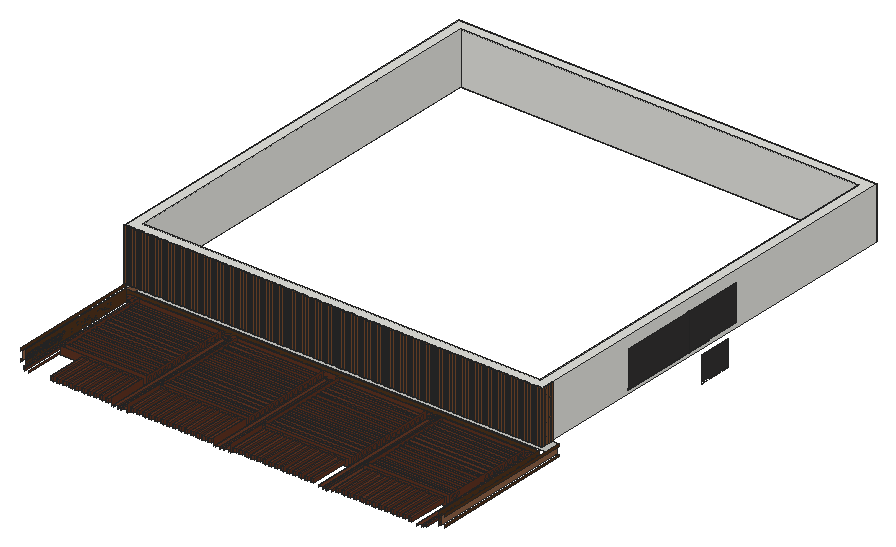
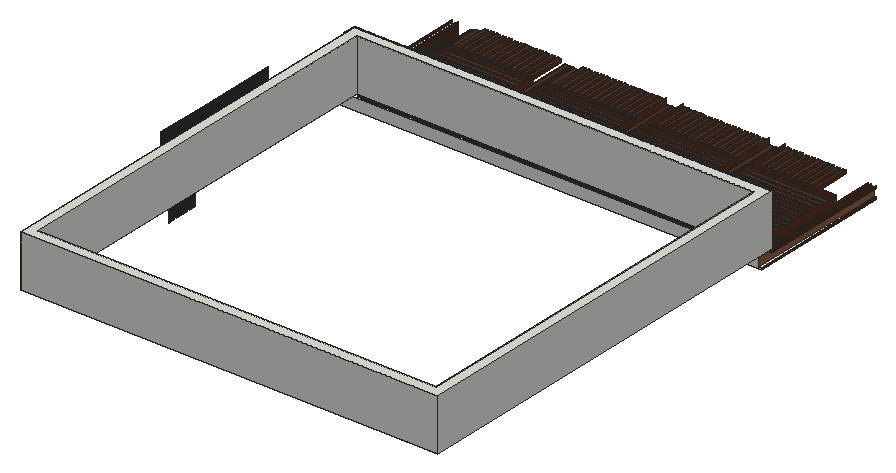
# SketchUp Ruby script. Lengths in inches.
U = 1.inch
M = Sketchup.active_model
def pt(a) = Geom::Point3d.new(a.map { |v| v * U })
def face(e, loops, mat)
  f = e.add_face(loops[0].map { |a| pt(a) })
  loops[1..].each { |l| e.add_face(l.map { |a| pt(a) }).erase! }
  f.material = f.back_material = mat if mat
  f
end
# faces: each face lists its corners as indices into pts; further lists are holes
def faces(e, pts, list, mat = nil) = list.each { |f| face(e, (f[0].is_a?(Array) ? f : [f]).map { |l| l.map { |i| pts[i] } }, mat) }
# xy, xz, yz: faces in a plane at the given z, y or x. An outline is a flat list of corners, or four numbers for a rectangle; further outlines are holes
def ring(l) = l.size == 4 ? [[l[0], l[1]], [l[2], l[1]], [l[2], l[3]], [l[0], l[3]]] : l.each_slice(2).to_a
def flat(e, list, mat, &to3) = list.each { |f| face(e, (f[0].is_a?(Array) ? f : [f]).map { |l| ring(l).map { |u, v| to3.(u, v) } }, mat) }
def xy(e, z, list, mat = nil) = flat(e, list, mat) { |x, y| [x, y, z] }
def xz(e, y, list, mat = nil) = flat(e, list, mat) { |x, z| [x, y, z] }
def yz(e, x, list, mat = nil) = flat(e, list, mat) { |y, z| [x, y, z] }
def lines(e, pts, list) = list.each { |a, b| e.add_line(pt(pts[a]), pt(pts[b])) }
# prism: a flat outline (further loops are holes) pulled along v
def prism(e, loops, v, mat = nil)
  f = face(e, loops, mat); d = Geom::Vector3d.new(v.map { |x| x * U })
  f.pushpull(f.normal.samedirection?(d) ? d.length : -d.length)
end
def box(e, o, s, mat = nil) = prism(e, [[o, [o[0] + s[0], o[1], o[2]], [o[0] + s[0], o[1] + s[1], o[2]], [o[0], o[1] + s[1], o[2]]]], [0, 0, s[2]], mat)
def at(x, y, z, deg = 0) = Geom::Transformation.translation(pt([x, y, z])) * Geom::Transformation.rotation(ORIGIN, Z_AXIS, deg.degrees)
def axes(o, x, y, z) = Geom::Transformation.new([*x, 0, *y, 0, *z, 0, *pt(o).to_a, 1])
def part(name) = M.definitions.add(name)
# library, detail: a bought-in or finely detailed component or shape, given as its bounding box
def library(name, o, s) = part(name).tap { |d| box(d.entities, o, s) }
def detail(e, o, s) = box(e.add_group.entities, o, s)
def put(e, d, t, mat = nil) = e.add_instance(d, t).tap { |i| i.material = mat if mat }
def group(e, t, mat = nil) = e.add_group.tap { |g| g.transformation = t; g.material = mat if mat }.entities
root = M.entities
M.materials.add("1799 AP 8574 BURNISHED CARAMEL").color = [140, 96, 69]
M.materials.add("1816 AP K197 Dark Kaapi-N").color = [79, 50, 27]
M.materials.add("[Granite Dark Gray]").color = [51, 50, 50]
M.materials.add("[Wood Cherry Original]").color = [118, 74, 44]
M.materials.add("[Wood Cherry Original]1").color = [93, 50, 33]
c1 = part("3")
box(c1.entities,[0,0,0],[3,2,36])
c2 = part("2")
box(c2.entities,[0,0,0],[3,2,75.23])
c3 = part("Group247\#1")
box(c3.entities,[-192,-24,0],[2.5,48,0.5])
c4 = part("Group248\#1")
box(c4.entities,[-189,-24,0],[2.5,48,0.5])
c5 = part("Group249\#1")
box(c5.entities,[-186,-24,0],[2.5,48,0.5])
c6 = part("Group250\#1")
box(c6.entities,[-183,-24,0],[2.5,48,0.5])
c7 = part("Group251\#1")
box(c7.entities,[-180,-24,0],[2.5,48,0.5])
c8 = part("Group252\#1")
box(c8.entities,[-177,-24,0],[2.5,48,0.5])
c9 = part("Group253\#1")
box(c9.entities,[-174,-24,0],[2.5,48,0.5])
c10 = part("Group254\#1")
box(c10.entities,[-171,-24,0],[2.5,48,0.5])
c11 = part("Group255\#1")
box(c11.entities,[-168,-24,0],[2.5,48,0.5])
c12 = part("Group256\#1")
box(c12.entities,[-165,-24,0],[2.5,48,0.5])
c13 = part("Group257\#1")
box(c13.entities,[-162,-24,0],[2.5,48,0.5])
c14 = part("Group258\#1")
box(c14.entities,[-159,-24,0],[2.5,48,0.5])
c15 = part("Group259\#1")
box(c15.entities,[-156,-24,0],[2.5,48,0.5])
c16 = part("Group260\#1")
box(c16.entities,[-153,-24,0],[2.5,48,0.5])
c17 = part("Group261\#1")
box(c17.entities,[-150,-24,0],[2.5,48,0.5])
c18 = part("Group262\#1")
box(c18.entities,[-147,-24,0],[2.5,48,0.5])
c19 = part("Group263\#1")
box(c19.entities,[-144,-24,0],[2.5,48,0.5])
c20 = part("Group264\#1")
box(c20.entities,[-141,-24,0],[2.5,48,0.5])
c21 = part("Group265\#1")
box(c21.entities,[-138,-24,0],[2.5,48,0.5])
c22 = part("Group266\#1")
box(c22.entities,[-135,-24,0],[2.5,48,0.5])
c23 = part("Group267\#1")
box(c23.entities,[-132,-24,0],[2.5,48,0.5])
c24 = part("Group268\#1")
box(c24.entities,[-129,-24,0],[2.5,48,0.5])
c25 = part("Group269\#1")
box(c25.entities,[-126,-24,0],[2.5,48,0.5])
c26 = part("Group270\#1")
box(c26.entities,[-123,-24,0],[2.5,48,0.5])
c27 = part("Group271\#1")
box(c27.entities,[-120,-24,0],[2.5,48,0.5])
c28 = part("Group272\#1")
box(c28.entities,[-117,-24,0],[2.5,48,0.5])
c29 = part("Group273\#1")
box(c29.entities,[-114,-24,0],[2.5,48,0.5])
c30 = part("Group274\#1")
box(c30.entities,[-111,-24,0],[2.5,48,0.5])
c31 = part("Group275\#1")
box(c31.entities,[-108,-24,0],[2.5,48,0.5])
c32 = part("Group276\#1")
box(c32.entities,[-105,-24,0],[2.5,48,0.5])
c33 = part("Group277\#1")
box(c33.entities,[-102,-24,0],[2.5,48,0.5])
c34 = part("Group278\#1")
box(c34.entities,[-99,-24,0],[2.5,48,0.5])
c35 = part("Group279\#1")
box(c35.entities,[-96,-24,0],[2.5,48,0.5])
c36 = part("Group280\#1")
box(c36.entities,[-93,-24,0],[2.5,48,0.5])
c37 = part("Group281\#1")
box(c37.entities,[-90,-24,0],[2.5,48,0.5])
c38 = part("Group282\#1")
box(c38.entities,[-87,-24,0],[2.5,48,0.5])
c39 = part("Group283\#1")
box(c39.entities,[-84,-24,0],[2.5,48,0.5])
c40 = part("Group284\#1")
box(c40.entities,[-81,-24,0],[2.5,48,0.5])
c41 = part("Group285\#1")
box(c41.entities,[-78,-24,0],[2.5,48,0.5])
c42 = part("Group286\#1")
box(c42.entities,[-75,-24,0],[2.5,48,0.5])
c43 = part("Group287\#1")
box(c43.entities,[-72,-24,0],[2.5,48,0.5])
c44 = part("Group288\#1")
box(c44.entities,[-69,-24,0],[2.5,48,0.5])
c45 = part("Group289\#1")
box(c45.entities,[-66,-24,0],[2.5,48,0.5])
c46 = part("Group290\#1")
box(c46.entities,[-63,-24,0],[2.5,48,0.5])
c47 = part("Group291\#1")
box(c47.entities,[-60,-24,0],[2.5,48,0.5])
c48 = part("Group292\#1")
box(c48.entities,[-57,-24,0],[2.5,48,0.5])
c49 = part("Group293\#1")
box(c49.entities,[-54,-24,0],[2.5,48,0.5])
c50 = part("Group294\#1")
box(c50.entities,[-51,-24,0],[2.5,48,0.5])
c51 = part("Group295\#1")
box(c51.entities,[-48,-24,0],[2.5,48,0.5])
c52 = part("Group296\#1")
box(c52.entities,[-45,-24,0],[2.5,48,0.5])
c53 = part("Group297\#1")
box(c53.entities,[-42,-24,0],[2.5,48,0.5])
c54 = part("Group298\#1")
box(c54.entities,[-39,-24,0],[2.5,48,0.5])
c55 = part("Group299\#1")
box(c55.entities,[-36,-24,0],[2.5,48,0.5])
c56 = part("Group300\#1")
box(c56.entities,[-33,-24,0],[2.5,48,0.5])
c57 = part("Group301\#1")
box(c57.entities,[-30,-24,0],[2.5,48,0.5])
c58 = part("Group302\#1")
box(c58.entities,[-27,-24,0],[2.5,48,0.5])
c59 = part("Group303\#1")
box(c59.entities,[-24,-24,0],[2.5,48,0.5])
c60 = part("Group304\#1")
box(c60.entities,[-21,-24,0],[2.5,48,0.5])
c61 = part("Group305\#1")
box(c61.entities,[-18,-24,0],[2.5,48,0.5])
c62 = part("Group306\#1")
box(c62.entities,[-15,-24,0],[2.5,48,0.5])
c63 = part("Group307\#1")
box(c63.entities,[-12,-24,0],[2.5,48,0.5])
c64 = part("Group308\#1")
box(c64.entities,[-9,-24,0],[2.5,48,0.5])
c65 = part("Group309\#1")
box(c65.entities,[-6,-24,0],[2.5,48,0.5])
c66 = part("Group310\#1")
box(c66.entities,[-3,-24,0],[2.5,48,0.5])
c67 = part("Group311\#1")
box(c67.entities,[0,-24,0],[2.5,48,0.5])
c68 = part("Group312\#1")
box(c68.entities,[3,-24,0],[2.5,48,0.5])
c69 = part("Group313\#1")
box(c69.entities,[6,-24,0],[2.5,48,0.5])
c70 = part("Group314\#1")
box(c70.entities,[9,-24,0],[2.5,48,0.5])
c71 = part("Group315\#1")
box(c71.entities,[12,-24,0],[2.5,48,0.5])
c72 = part("Group316\#1")
box(c72.entities,[15,-24,0],[2.5,48,0.5])
c73 = part("Group317\#1")
box(c73.entities,[18,-24,0],[2.5,48,0.5])
c74 = part("Group318\#1")
box(c74.entities,[21,-24,0],[2.5,48,0.5])
c75 = part("Group319\#1")
box(c75.entities,[24,-24,0],[2.5,48,0.5])
c76 = part("Group320\#1")
box(c76.entities,[27,-24,0],[2.5,48,0.5])
c77 = part("Group321\#1")
box(c77.entities,[30,-24,0],[2.5,48,0.5])
c78 = part("Group322\#1")
box(c78.entities,[33,-24,0],[2.5,48,0.5])
c79 = part("Group323\#1")
box(c79.entities,[36,-24,0],[2.5,48,0.5])
c80 = part("Group324\#1")
box(c80.entities,[39,-24,0],[2.5,48,0.5])
c81 = part("Group325\#1")
box(c81.entities,[42,-24,0],[2.5,48,0.5])
c82 = part("Group326\#1")
box(c82.entities,[45,-24,0],[2.5,48,0.5])
c83 = part("Group327\#1")
box(c83.entities,[48,-24,0],[2.5,48,0.5])
c84 = part("Group328\#1")
box(c84.entities,[51,-24,0],[2.5,48,0.5])
c85 = part("Group329\#1")
box(c85.entities,[54,-24,0],[2.5,48,0.5])
c86 = part("Group330\#1")
box(c86.entities,[57,-24,0],[2.5,48,0.5])
c87 = part("Group331\#1")
box(c87.entities,[60,-24,0],[2.5,48,0.5])
c88 = part("Group332\#1")
box(c88.entities,[63,-24,0],[2.5,48,0.5])
c89 = part("Group333\#1")
box(c89.entities,[66,-24,0],[2.5,48,0.5])
c90 = part("Group334\#1")
box(c90.entities,[69,-24,0],[2.5,48,0.5])
c91 = part("Group335\#1")
box(c91.entities,[72,-24,0],[2.5,48,0.5])
c92 = part("Group336\#1")
box(c92.entities,[75,-24,0],[2.5,48,0.5])
c93 = part("Group337\#1")
box(c93.entities,[78,-24,0],[2.5,48,0.5])
c94 = part("Group338\#1")
box(c94.entities,[81,-24,0],[2.5,48,0.5])
c95 = part("Group339\#1")
box(c95.entities,[84,-24,0],[2.5,48,0.5])
c96 = part("Group340\#1")
box(c96.entities,[87,-24,0],[2.5,48,0.5])
c97 = part("Group341\#1")
box(c97.entities,[90,-24,0],[2.5,48,0.5])
c98 = part("Group342\#1")
box(c98.entities,[93,-24,0],[2.5,48,0.5])
c99 = part("Group343\#1")
box(c99.entities,[96,-24,0],[2.5,48,0.5])
c100 = part("Group344\#1")
box(c100.entities,[99,-24,0],[2.5,48,0.5])
c101 = part("Group345\#1")
box(c101.entities,[102,-24,0],[2.5,48,0.5])
c102 = part("Group346\#1")
box(c102.entities,[105,-24,0],[2.5,48,0.5])
c103 = part("Group347\#1")
box(c103.entities,[108,-24,0],[2.5,48,0.5])
c104 = part("Group348\#1")
box(c104.entities,[111,-24,0],[2.5,48,0.5])
c105 = part("Group349\#1")
box(c105.entities,[114,-24,0],[2.5,48,0.5])
c106 = part("Group350\#1")
box(c106.entities,[117,-24,0],[2.5,48,0.5])
c107 = part("Group351\#1")
box(c107.entities,[120,-24,0],[2.5,48,0.5])
c108 = part("Group352\#1")
box(c108.entities,[123,-24,0],[2.5,48,0.5])
c109 = part("Group353\#1")
box(c109.entities,[126,-24,0],[2.5,48,0.5])
c110 = part("Group354\#1")
box(c110.entities,[129,-24,0],[2.5,48,0.5])
c111 = part("Group355\#1")
box(c111.entities,[132,-24,0],[2.5,48,0.5])
c112 = part("Group356\#1")
box(c112.entities,[135,-24,0],[2.5,48,0.5])
c113 = part("Group357\#1")
box(c113.entities,[138,-24,0],[2.5,48,0.5])
c114 = part("Group358\#1")
box(c114.entities,[141,-24,0],[2.5,48,0.5])
c115 = part("Group359\#1")
box(c115.entities,[144,-24,0],[2.5,48,0.5])
c116 = part("Group360\#1")
box(c116.entities,[147,-24,0],[2.5,48,0.5])
c117 = part("Group361\#1")
box(c117.entities,[150,-24,0],[2.5,48,0.5])
c118 = part("Group362\#1")
box(c118.entities,[153,-24,0],[2.5,48,0.5])
c119 = part("Group363\#1")
box(c119.entities,[156,-24,0],[2.5,48,0.5])
c120 = part("Group364\#1")
box(c120.entities,[159,-24,0],[2.5,48,0.5])
c121 = part("Group365\#1")
box(c121.entities,[162,-24,0],[2.5,48,0.5])
c122 = part("Group366\#1")
box(c122.entities,[165,-24,0],[2.5,48,0.5])
c123 = part("Group367\#1")
box(c123.entities,[168,-24,0],[2.5,48,0.5])
c124 = part("Group368\#1")
box(c124.entities,[171,-24,0],[2.5,48,0.5])
c125 = part("Group369\#1")
box(c125.entities,[174,-24,0],[2.5,48,0.5])
c126 = part("Group370\#1")
box(c126.entities,[177,-24,0],[2.5,48,0.5])
c127 = part("Group371\#1")
box(c127.entities,[180,-24,0],[2.5,48,0.5])
c128 = part("Group372\#1")
box(c128.entities,[183,-24,0],[2.5,48,0.5])
c129 = part("Group373\#1")
box(c129.entities,[186,-24,0],[2.5,48,0.5])
c130 = part("Group374\#1")
box(c130.entities,[189,-24,0],[2.5,48,0.5])
c131 = part("Group245\#1")
put(c131.entities,c3,at(0,0,0))
put(c131.entities,c4,at(0,0,0))
put(c131.entities,c5,at(0,0,0))
put(c131.entities,c6,at(0,0,0))
put(c131.entities,c7,at(0,0,0))
put(c131.entities,c8,at(0,0,0))
put(c131.entities,c9,at(0,0,0))
put(c131.entities,c10,at(0,0,0))
put(c131.entities,c11,at(0,0,0))
put(c131.entities,c12,at(0,0,0))
put(c131.entities,c13,at(0,0,0))
put(c131.entities,c14,at(0,0,0))
put(c131.entities,c15,at(0,0,0))
put(c131.entities,c16,at(0,0,0))
put(c131.entities,c17,at(0,0,0))
put(c131.entities,c18,at(0,0,0))
put(c131.entities,c19,at(0,0,0))
put(c131.entities,c20,at(0,0,0))
put(c131.entities,c21,at(0,0,0))
put(c131.entities,c22,at(0,0,0))
put(c131.entities,c23,at(0,0,0))
put(c131.entities,c24,at(0,0,0))
put(c131.entities,c25,at(0,0,0))
put(c131.entities,c26,at(0,0,0))
put(c131.entities,c27,at(0,0,0))
put(c131.entities,c28,at(0,0,0))
put(c131.entities,c29,at(0,0,0))
put(c131.entities,c30,at(0,0,0))
put(c131.entities,c31,at(0,0,0))
put(c131.entities,c32,at(0,0,0))
put(c131.entities,c33,at(0,0,0))
put(c131.entities,c34,at(0,0,0))
put(c131.entities,c35,at(0,0,0))
put(c131.entities,c36,at(0,0,0))
put(c131.entities,c37,at(0,0,0))
put(c131.entities,c38,at(0,0,0))
put(c131.entities,c39,at(0,0,0))
put(c131.entities,c40,at(0,0,0))
put(c131.entities,c41,at(0,0,0))
put(c131.entities,c42,at(0,0,0))
put(c131.entities,c43,at(0,0,0))
put(c131.entities,c44,at(0,0,0))
put(c131.entities,c45,at(0,0,0))
put(c131.entities,c46,at(0,0,0))
put(c131.entities,c47,at(0,0,0))
put(c131.entities,c48,at(0,0,0))
put(c131.entities,c49,at(0,0,0))
put(c131.entities,c50,at(0,0,0))
put(c131.entities,c51,at(0,0,0))
put(c131.entities,c52,at(0,0,0))
put(c131.entities,c53,at(0,0,0))
put(c131.entities,c54,at(0,0,0))
put(c131.entities,c55,at(0,0,0))
put(c131.entities,c56,at(0,0,0))
put(c131.entities,c57,at(0,0,0))
put(c131.entities,c58,at(0,0,0))
put(c131.entities,c59,at(0,0,0))
put(c131.entities,c60,at(0,0,0))
put(c131.entities,c61,at(0,0,0))
put(c131.entities,c62,at(0,0,0))
put(c131.entities,c63,at(0,0,0))
put(c131.entities,c64,at(0,0,0))
put(c131.entities,c65,at(0,0,0))
put(c131.entities,c66,at(0,0,0))
put(c131.entities,c67,at(0,0,0))
put(c131.entities,c68,at(0,0,0))
put(c131.entities,c69,at(0,0,0))
put(c131.entities,c70,at(0,0,0))
put(c131.entities,c71,at(0,0,0))
put(c131.entities,c72,at(0,0,0))
put(c131.entities,c73,at(0,0,0))
put(c131.entities,c74,at(0,0,0))
put(c131.entities,c75,at(0,0,0))
put(c131.entities,c76,at(0,0,0))
put(c131.entities,c77,at(0,0,0))
put(c131.entities,c78,at(0,0,0))
put(c131.entities,c79,at(0,0,0))
put(c131.entities,c80,at(0,0,0))
put(c131.entities,c81,at(0,0,0))
put(c131.entities,c82,at(0,0,0))
put(c131.entities,c83,at(0,0,0))
put(c131.entities,c84,at(0,0,0))
put(c131.entities,c85,at(0,0,0))
put(c131.entities,c86,at(0,0,0))
put(c131.entities,c87,at(0,0,0))
put(c131.entities,c88,at(0,0,0))
put(c131.entities,c89,at(0,0,0))
put(c131.entities,c90,at(0,0,0))
put(c131.entities,c91,at(0,0,0))
put(c131.entities,c92,at(0,0,0))
put(c131.entities,c93,at(0,0,0))
put(c131.entities,c94,at(0,0,0))
put(c131.entities,c95,at(0,0,0))
put(c131.entities,c96,at(0,0,0))
put(c131.entities,c97,at(0,0,0))
put(c131.entities,c98,at(0,0,0))
put(c131.entities,c99,at(0,0,0))
put(c131.entities,c100,at(0,0,0))
put(c131.entities,c101,at(0,0,0))
put(c131.entities,c102,at(0,0,0))
put(c131.entities,c103,at(0,0,0))
put(c131.entities,c104,at(0,0,0))
put(c131.entities,c105,at(0,0,0))
put(c131.entities,c106,at(0,0,0))
put(c131.entities,c107,at(0,0,0))
put(c131.entities,c108,at(0,0,0))
put(c131.entities,c109,at(0,0,0))
put(c131.entities,c110,at(0,0,0))
put(c131.entities,c111,at(0,0,0))
put(c131.entities,c112,at(0,0,0))
put(c131.entities,c113,at(0,0,0))
put(c131.entities,c114,at(0,0,0))
put(c131.entities,c115,at(0,0,0))
put(c131.entities,c116,at(0,0,0))
put(c131.entities,c117,at(0,0,0))
put(c131.entities,c118,at(0,0,0))
put(c131.entities,c119,at(0,0,0))
put(c131.entities,c120,at(0,0,0))
put(c131.entities,c121,at(0,0,0))
put(c131.entities,c122,at(0,0,0))
put(c131.entities,c123,at(0,0,0))
put(c131.entities,c124,at(0,0,0))
put(c131.entities,c125,at(0,0,0))
put(c131.entities,c126,at(0,0,0))
put(c131.entities,c127,at(0,0,0))
put(c131.entities,c128,at(0,0,0))
put(c131.entities,c129,at(0,0,0))
put(c131.entities,c130,at(0,0,0))
c132 = part("Group384\#1")
box(c132.entities,[-6,-24,0],[1.5,48,0.5])
c133 = part("Group385\#1")
box(c133.entities,[-4,-24,0],[1.5,48,0.5])
c134 = part("Group386\#1")
box(c134.entities,[-2,-24,0],[1.5,48,0.5])
c135 = part("Group387\#1")
box(c135.entities,[0,-24,0],[1.5,48,0.5])
c136 = part("Group388\#1")
box(c136.entities,[2,-24,0],[1.5,48,0.5])
c137 = part("Group389\#1")
box(c137.entities,[4,-24,0],[1.5,48,0.5])
c138 = part("Group382\#1")
put(c138.entities,c132,at(0,0,0))
put(c138.entities,c133,at(0,0,0))
put(c138.entities,c134,at(0,0,0))
put(c138.entities,c135,at(0,0,0))
put(c138.entities,c136,at(0,0,0))
put(c138.entities,c137,at(0,0,0))
xy(root,378,[[436.875,393,437,423]],"[Granite Dark Gray]")
xy(root,392.75,[[142.75,84.5,146.75,209.5],[147.75,84.5,149.75,209.5],[150.75,84.5,154.75,209.5],[237,84.5,241,209.5],[242,84.5,244,209.5],
  [245,84.5,249,209.5],[331.25,84.5,335.25,209.5],[336.25,84.5,338.25,209.5],[339.25,84.5,343.25,209.5],[421.48,84.6,421.48,209.5,425.48,209.5,425.48,85.9,425.32,85.81,424.92,85.61,424.51,85.43,424.09,85.26,423.67,85.11,423.24,84.97,422.8,84.85,422.37,84.75,421.92,84.66,421.5,84.6],
  [59.52,86.5,59.49,86.52,59.24,86.7,58.88,86.97,58.42,87.35,58.19,87.56,58.08,87.66,57.66,88.08,57.52,88.23,57.52,209.5,59.52,209.5],[426.48,86.5,426.48,209.5,428.48,209.5,428.48,88.23,428.34,88.08,428.02,87.76,427.81,87.56,427.69,87.45,427.47,87.26,427.35,87.16,427.12,86.97,426.64,86.61,426.51,86.52]],"[Wood Cherry Original]1")
xy(root,416,[[443.875,300,444,363],[443.875,363,444,369],[443.875,370,444,393]],"[Granite Dark Gray]")
xy(root,417,[[443.875,300,444,363],[443.875,363,444,369],[443.875,370,444,393]],"[Granite Dark Gray]")
xz(root,120.5,[[66.02,391,141.25,398],[156.25,391,235.5,398],[250.5,391,329.75,398],[344.75,391,419.98,398]],"[Wood Cherry Original]1")
xz(root,124.5,[[66.02,391,141.25,398],[156.25,391,235.5,398],[250.5,391,329.75,398],[344.75,391,419.98,398]],"[Wood Cherry Original]1")
xz(root,209.5,[[57.52,391,59.52,392.75],[60.52,391,64.52,392.75],[66.02,391,141.25,398],[142.75,391,146.75,392.75],[147.75,391,149.75,392.75],
  [150.75,391,154.75,392.75],[156.25,391,235.5,398],[237,391,241,392.75],[242,391,244,392.75],[245,391,249,392.75],
  [250.5,391,329.75,398],[331.25,391,335.25,392.75],[336.25,391,338.25,392.75],[339.25,391,343.25,392.75],[344.75,391,419.98,398],
  [421.48,391,425.48,392.75],[426.48,391,428.48,392.75]],"[Wood Cherry Original]1")
xz(root,211,[[53,390,433,401]],"1816 AP K197 Dark Kaapi-N")
xz(root,211,[[53,391,433,398]],"[Wood Cherry Original]1")
xz(root,216,[[48,399,50,401]])
xz(root,228,[[48,390,48,392,50,392,50,401,438,401,438,399,436,399,436,392,438,392,438,390]])
xz(root,369,[[443.875,417,444,450]],"[Granite Dark Gray]")
xz(root,370,[[443.875,417,444,450]],"[Granite Dark Gray]")
yz(root,48,[[96,390,228,392],[96,399,216,401]],"1816 AP K197 Dark Kaapi-N")
yz(root,50,[[216,399,228,401]])
yz(root,50,[[96.01,392,228,399]],"1799 AP 8574 BURNISHED CARAMEL")
yz(root,53,[[96.02,390,211,401]],"1816 AP K197 Dark Kaapi-N")
yz(root,53,[[96.02,391,211,398]],"[Wood Cherry Original]1")
yz(root,57.52,[[88.23,391,209.5,392.75]],"[Wood Cherry Original]1")
yz(root,59.52,[[86.5,391,209.5,392.75]],"[Wood Cherry Original]1")
yz(root,60.52,[[85.9,391,209.5,392.75]],"[Wood Cherry Original]1")
yz(root,64.52,[[84.61,391,209.5,392.75]],"[Wood Cherry Original]1")
yz(root,66.02,[[124.5,391,209.5,398]],"[Wood Cherry Original]1")
yz(root,141.25,[[84.5,391,120.5,398],[124.5,391,209.5,398]],"[Wood Cherry Original]1")
yz(root,142.75,[[84.5,391,209.5,392.75]],"[Wood Cherry Original]1")
yz(root,146.75,[[84.5,391,209.5,392.75]],"[Wood Cherry Original]1")
yz(root,147.75,[[84.5,391,209.5,392.75]],"[Wood Cherry Original]1")
yz(root,149.75,[[84.5,391,209.5,392.75]],"[Wood Cherry Original]1")
yz(root,150.75,[[84.5,391,209.5,392.75]],"[Wood Cherry Original]1")
yz(root,154.75,[[84.5,391,209.5,392.75]],"[Wood Cherry Original]1")
yz(root,156.25,[[84.5,391,120.5,398],[124.5,391,209.5,398]],"[Wood Cherry Original]1")
yz(root,235.5,[[84.5,391,120.5,398],[124.5,391,209.5,398]],"[Wood Cherry Original]1")
yz(root,237,[[84.5,391,209.5,392.75]],"[Wood Cherry Original]1")
yz(root,241,[[84.5,391,209.5,392.75]],"[Wood Cherry Original]1")
yz(root,242,[[84.5,391,209.5,392.75]],"[Wood Cherry Original]1")
yz(root,244,[[84.5,391,209.5,392.75]],"[Wood Cherry Original]1")
yz(root,245,[[84.5,391,209.5,392.75]],"[Wood Cherry Original]1")
yz(root,249,[[84.5,391,209.5,392.75]],"[Wood Cherry Original]1")
yz(root,250.5,[[84.5,391,120.5,398],[124.5,391,209.5,398]],"[Wood Cherry Original]1")
yz(root,329.75,[[124.5,391,209.5,398]],"[Wood Cherry Original]1")
yz(root,331.25,[[84.5,391,209.5,392.75]],"[Wood Cherry Original]1")
yz(root,335.25,[[84.5,391,209.5,392.75]],"[Wood Cherry Original]1")
yz(root,336.25,[[84.5,391,209.5,392.75]],"[Wood Cherry Original]1")
yz(root,338.25,[[84.5,391,209.5,392.75]],"[Wood Cherry Original]1")
yz(root,339.25,[[84.5,391,209.5,392.75]],"[Wood Cherry Original]1")
yz(root,343.25,[[84.5,391,209.5,392.75]],"[Wood Cherry Original]1")
yz(root,344.75,[[124.5,391,209.5,398]],"[Wood Cherry Original]1")
yz(root,419.98,[[124.5,391,209.5,398]],"[Wood Cherry Original]1")
yz(root,421.48,[[84.6,391,209.5,392.75]],"[Wood Cherry Original]1")
yz(root,425.48,[[85.9,391,209.5,392.75]],"[Wood Cherry Original]1")
yz(root,426.48,[[86.5,391,209.5,392.75]],"[Wood Cherry Original]1")
yz(root,428.48,[[88.23,391,209.5,392.75]],"[Wood Cherry Original]1")
yz(root,433,[[96.02,390,211,401]],"1816 AP K197 Dark Kaapi-N")
yz(root,433,[[96.02,391,211,398]],"[Wood Cherry Original]1")
yz(root,436,[[96.01,392,228,399]],"1799 AP 8574 BURNISHED CARAMEL")
yz(root,437,[[393,379,423,402]],"[Granite Dark Gray]")
yz(root,438,[[96,390,228,392],[96,399,228,401]],"1816 AP K197 Dark Kaapi-N")
yz(root,444,[[300,417,369,450],[370,417,423,450]],"[Granite Dark Gray]")
p = [[432,216,400.98],[432,216,390],[54.5,120.5,391],[54.5,120.5,398]]
lines(root,p,[[0,1],[2,3]])
put(root,c1,axes([85.33,120.5,392.75],[1,0,0],[0,0,1.75],[0,-1,0]),"[Wood Cherry Original]1")
put(root,c1,axes([90.93,120.5,392.75],[1,0,0],[0,0,1.75],[0,-1,0]),"[Wood Cherry Original]1")
put(root,c1,axes([96.53,120.5,392.75],[1,0,0],[0,0,1.75],[0,-1,0]),"[Wood Cherry Original]1")
put(root,c1,axes([102.14,120.5,392.75],[1,0,0],[0,0,1.75],[0,-1,0]),"[Wood Cherry Original]1")
put(root,c1,axes([107.74,120.5,392.75],[1,0,0],[0,0,1.75],[0,-1,0]),"[Wood Cherry Original]1")
put(root,c1,axes([113.34,120.5,392.75],[1,0,0],[0,0,1.75],[0,-1,0]),"[Wood Cherry Original]1")
put(root,c1,axes([118.94,120.5,392.75],[1,0,0],[0,0,1.75],[0,-1,0]),"[Wood Cherry Original]1")
put(root,c1,axes([124.55,120.5,392.75],[1,0,0],[0,0,1.75],[0,-1,0]),"[Wood Cherry Original]1")
put(root,c1,axes([130.15,120.5,392.75],[1,0,0],[0,0,1.75],[0,-1,0]),"[Wood Cherry Original]1")
put(root,c1,axes([135.75,120.5,392.75],[1,0,0],[0,0,1.75],[0,-1,0]),"[Wood Cherry Original]1")
put(root,c1,axes([158.75,120.5,392.75],[1,0,0],[0,0,1.75],[0,-1,0]),"[Wood Cherry Original]1")
put(root,c1,axes([164.23,120.5,392.75],[1,0,0],[0,0,1.75],[0,-1,0]),"[Wood Cherry Original]1")
put(root,c1,axes([169.71,120.5,392.75],[1,0,0],[0,0,1.75],[0,-1,0]),"[Wood Cherry Original]1")
put(root,c1,axes([175.19,120.5,392.75],[1,0,0],[0,0,1.75],[0,-1,0]),"[Wood Cherry Original]1")
put(root,c1,axes([180.67,120.5,392.75],[1,0,0],[0,0,1.75],[0,-1,0]),"[Wood Cherry Original]1")
put(root,c1,axes([186.15,120.5,392.75],[1,0,0],[0,0,1.75],[0,-1,0]),"[Wood Cherry Original]1")
put(root,c1,axes([191.63,120.5,392.75],[1,0,0],[0,0,1.75],[0,-1,0]),"[Wood Cherry Original]1")
put(root,c1,axes([197.12,120.5,392.75],[1,0,0],[0,0,1.75],[0,-1,0]),"[Wood Cherry Original]1")
put(root,c1,axes([202.6,120.5,392.75],[1,0,0],[0,0,1.75],[0,-1,0]),"[Wood Cherry Original]1")
put(root,c1,axes([208.08,120.5,392.75],[1,0,0],[0,0,1.75],[0,-1,0]),"[Wood Cherry Original]1")
put(root,c1,axes([213.56,120.5,392.75],[1,0,0],[0,0,1.75],[0,-1,0]),"[Wood Cherry Original]1")
put(root,c1,axes([219.04,120.5,392.75],[1,0,0],[0,0,1.75],[0,-1,0]),"[Wood Cherry Original]1")
put(root,c1,axes([224.52,120.5,392.75],[1,0,0],[0,0,1.75],[0,-1,0]),"[Wood Cherry Original]1")
put(root,c1,axes([230,120.5,392.75],[1,0,0],[0,0,1.75],[0,-1,0]),"[Wood Cherry Original]1")
put(root,c1,axes([352.85,120.5,392.75],[1,0,0],[0,0,1.75],[0,-1,0]),"[Wood Cherry Original]1")
put(root,c1,axes([369.66,120.5,392.75],[1,0,0],[0,0,1.75],[0,-1,0]),"[Wood Cherry Original]1")
put(root,c1,axes([364.06,120.5,392.75],[1,0,0],[0,0,1.75],[0,-1,0]),"[Wood Cherry Original]1")
put(root,c1,axes([358.45,120.5,392.75],[1,0,0],[0,0,1.75],[0,-1,0]),"[Wood Cherry Original]1")
put(root,c1,axes([347.25,120.5,392.75],[1,0,0],[0,0,1.75],[0,-1,0]),"[Wood Cherry Original]1")
put(root,c1,axes([414.48,120.5,392.75],[1,0,0],[0,0,1.75],[0,-1,0]),"[Wood Cherry Original]1")
put(root,c1,axes([392.07,120.5,392.75],[1,0,0],[0,0,1.75],[0,-1,0]),"[Wood Cherry Original]1")
put(root,c1,axes([397.67,120.5,392.75],[1,0,0],[0,0,1.75],[0,-1,0]),"[Wood Cherry Original]1")
put(root,c1,axes([375.26,120.5,392.75],[1,0,0],[0,0,1.75],[0,-1,0]),"[Wood Cherry Original]1")
put(root,c1,axes([380.86,120.5,392.75],[1,0,0],[0,0,1.75],[0,-1,0]),"[Wood Cherry Original]1")
put(root,c1,axes([403.27,120.5,392.75],[1,0,0],[0,0,1.75],[0,-1,0]),"[Wood Cherry Original]1")
put(root,c1,axes([386.47,120.5,392.75],[1,0,0],[0,0,1.75],[0,-1,0]),"[Wood Cherry Original]1")
put(root,c1,axes([408.875,120.5,392.75],[1,0,0],[0,0,1.75],[0,-1,0]),"[Wood Cherry Original]1")
put(root,c1,axes([280.4,120.5,392.75],[1,0,0],[0,0,1.75],[0,-1,0]),"[Wood Cherry Original]1")
put(root,c1,axes([253,120.5,392.75],[1,0,0],[0,0,1.75],[0,-1,0]),"[Wood Cherry Original]1")
put(root,c1,axes([269.44,120.5,392.75],[1,0,0],[0,0,1.75],[0,-1,0]),"[Wood Cherry Original]1")
put(root,c1,axes([274.92,120.5,392.75],[1,0,0],[0,0,1.75],[0,-1,0]),"[Wood Cherry Original]1")
put(root,c1,axes([263.96,120.5,392.75],[1,0,0],[0,0,1.75],[0,-1,0]),"[Wood Cherry Original]1")
put(root,c1,axes([258.48,120.5,392.75],[1,0,0],[0,0,1.75],[0,-1,0]),"[Wood Cherry Original]1")
put(root,c1,axes([285.88,120.5,392.75],[1,0,0],[0,0,1.75],[0,-1,0]),"[Wood Cherry Original]1")
put(root,c1,axes([291.37,120.5,392.75],[1,0,0],[0,0,1.75],[0,-1,0]),"[Wood Cherry Original]1")
put(root,c1,axes([313.29,120.5,392.75],[1,0,0],[0,0,1.75],[0,-1,0]),"[Wood Cherry Original]1")
put(root,c1,axes([318.77,120.5,392.75],[1,0,0],[0,0,1.75],[0,-1,0]),"[Wood Cherry Original]1")
put(root,c1,axes([324.25,120.5,392.75],[1,0,0],[0,0,1.75],[0,-1,0]),"[Wood Cherry Original]1")
put(root,c1,axes([302.33,120.5,392.75],[1,0,0],[0,0,1.75],[0,-1,0]),"[Wood Cherry Original]1")
put(root,c1,axes([296.85,120.5,392.75],[1,0,0],[0,0,1.75],[0,-1,0]),"[Wood Cherry Original]1")
put(root,c1,axes([307.81,120.5,392.75],[1,0,0],[0,0,1.75],[0,-1,0]),"[Wood Cherry Original]1")
put(root,c2,axes([344.75,127,392.75],[0,1,0],[0,0,1.75],[1,0,0]),"[Wood Cherry Original]1")
put(root,c2,axes([250.5,127,392.75],[0,1,0],[0,0,1.75],[1.05345,0,0]),"[Wood Cherry Original]1")
put(root,c2,axes([156.25,127,392.75],[0,1,0],[0,0,1.75],[1.05345,0,0]),"[Wood Cherry Original]1")
put(root,c2,axes([66.02,127,392.75],[0,1,0],[0,0,1.75],[1,0,0]),"[Wood Cherry Original]1")
put(root,c2,axes([344.75,132.5,392.75],[0,1,0],[0,0,1.75],[1,0,0]),"[Wood Cherry Original]1")
put(root,c2,axes([250.5,132.5,392.75],[0,1,0],[0,0,1.75],[1.05345,0,0]),"[Wood Cherry Original]1")
put(root,c2,axes([156.25,132.5,392.75],[0,1,0],[0,0,1.75],[1.05345,0,0]),"[Wood Cherry Original]1")
put(root,c2,axes([66.02,132.5,392.75],[0,1,0],[0,0,1.75],[1,0,0]),"[Wood Cherry Original]1")
put(root,c2,axes([344.75,138,392.75],[0,1,0],[0,0,1.75],[1,0,0]),"[Wood Cherry Original]1")
put(root,c2,axes([250.5,138,392.75],[0,1,0],[0,0,1.75],[1.05345,0,0]),"[Wood Cherry Original]1")
put(root,c2,axes([156.25,138,392.75],[0,1,0],[0,0,1.75],[1.05345,0,0]),"[Wood Cherry Original]1")
put(root,c2,axes([66.02,138,392.75],[0,1,0],[0,0,1.75],[1,0,0]),"[Wood Cherry Original]1")
put(root,c2,axes([344.75,143.5,392.75],[0,1,0],[0,0,1.75],[1,0,0]),"[Wood Cherry Original]1")
put(root,c2,axes([250.5,143.5,392.75],[0,1,0],[0,0,1.75],[1.05345,0,0]),"[Wood Cherry Original]1")
put(root,c2,axes([156.25,143.5,392.75],[0,1,0],[0,0,1.75],[1.05345,0,0]),"[Wood Cherry Original]1")
put(root,c2,axes([66.02,143.5,392.75],[0,1,0],[0,0,1.75],[1,0,0]),"[Wood Cherry Original]1")
put(root,c2,axes([344.75,149,392.75],[0,1,0],[0,0,1.75],[1,0,0]),"[Wood Cherry Original]1")
put(root,c2,axes([250.5,149,392.75],[0,1,0],[0,0,1.75],[1.05345,0,0]),"[Wood Cherry Original]1")
put(root,c2,axes([156.25,149,392.75],[0,1,0],[0,0,1.75],[1.05345,0,0]),"[Wood Cherry Original]1")
put(root,c2,axes([66.02,149,392.75],[0,1,0],[0,0,1.75],[1,0,0]),"[Wood Cherry Original]1")
put(root,c2,axes([344.75,154.5,392.75],[0,1,0],[0,0,1.75],[1,0,0]),"[Wood Cherry Original]1")
put(root,c2,axes([250.5,154.5,392.75],[0,1,0],[0,0,1.75],[1.05345,0,0]),"[Wood Cherry Original]1")
put(root,c2,axes([156.25,154.5,392.75],[0,1,0],[0,0,1.75],[1.05345,0,0]),"[Wood Cherry Original]1")
put(root,c2,axes([66.02,154.5,392.75],[0,1,0],[0,0,1.75],[1,0,0]),"[Wood Cherry Original]1")
put(root,c2,axes([344.75,160,392.75],[0,1,0],[0,0,1.75],[1,0,0]),"[Wood Cherry Original]1")
put(root,c2,axes([250.5,160,392.75],[0,1,0],[0,0,1.75],[1.05345,0,0]),"[Wood Cherry Original]1")
put(root,c2,axes([156.25,160,392.75],[0,1,0],[0,0,1.75],[1.05345,0,0]),"[Wood Cherry Original]1")
put(root,c2,axes([66.02,160,392.75],[0,1,0],[0,0,1.75],[1,0,0]),"[Wood Cherry Original]1")
put(root,c2,axes([344.75,165.5,392.75],[0,1,0],[0,0,1.75],[1,0,0]),"[Wood Cherry Original]1")
put(root,c2,axes([250.5,165.5,392.75],[0,1,0],[0,0,1.75],[1.05345,0,0]),"[Wood Cherry Original]1")
put(root,c2,axes([156.25,165.5,392.75],[0,1,0],[0,0,1.75],[1.05345,0,0]),"[Wood Cherry Original]1")
put(root,c2,axes([66.02,165.5,392.75],[0,1,0],[0,0,1.75],[1,0,0]),"[Wood Cherry Original]1")
put(root,c2,axes([344.75,171,392.75],[0,1,0],[0,0,1.75],[1,0,0]),"[Wood Cherry Original]1")
put(root,c2,axes([250.5,171,392.75],[0,1,0],[0,0,1.75],[1.05345,0,0]),"[Wood Cherry Original]1")
put(root,c2,axes([156.25,171,392.75],[0,1,0],[0,0,1.75],[1.05345,0,0]),"[Wood Cherry Original]1")
put(root,c2,axes([66.02,171,392.75],[0,1,0],[0,0,1.75],[1,0,0]),"[Wood Cherry Original]1")
put(root,c2,axes([344.75,176.5,392.75],[0,1,0],[0,0,1.75],[1,0,0]),"[Wood Cherry Original]1")
put(root,c2,axes([250.5,176.5,392.75],[0,1,0],[0,0,1.75],[1.05345,0,0]),"[Wood Cherry Original]1")
put(root,c2,axes([156.25,176.5,392.75],[0,1,0],[0,0,1.75],[1.05345,0,0]),"[Wood Cherry Original]1")
put(root,c2,axes([66.02,176.5,392.75],[0,1,0],[0,0,1.75],[1,0,0]),"[Wood Cherry Original]1")
put(root,c2,axes([344.75,182,392.75],[0,1,0],[0,0,1.75],[1,0,0]),"[Wood Cherry Original]1")
put(root,c2,axes([250.5,182,392.75],[0,1,0],[0,0,1.75],[1.05345,0,0]),"[Wood Cherry Original]1")
put(root,c2,axes([156.25,182,392.75],[0,1,0],[0,0,1.75],[1.05345,0,0]),"[Wood Cherry Original]1")
put(root,c2,axes([66.02,182,392.75],[0,1,0],[0,0,1.75],[1,0,0]),"[Wood Cherry Original]1")
put(root,c2,axes([344.75,187.5,392.75],[0,1,0],[0,0,1.75],[1,0,0]),"[Wood Cherry Original]1")
put(root,c2,axes([250.5,187.5,392.75],[0,1,0],[0,0,1.75],[1.05345,0,0]),"[Wood Cherry Original]1")
put(root,c2,axes([156.25,187.5,392.75],[0,1,0],[0,0,1.75],[1.05345,0,0]),"[Wood Cherry Original]1")
put(root,c2,axes([66.02,187.5,392.75],[0,1,0],[0,0,1.75],[1,0,0]),"[Wood Cherry Original]1")
put(root,c2,axes([344.75,193,392.75],[0,1,0],[0,0,1.75],[1,0,0]),"[Wood Cherry Original]1")
put(root,c2,axes([250.5,193,392.75],[0,1,0],[0,0,1.75],[1.05345,0,0]),"[Wood Cherry Original]1")
put(root,c2,axes([156.25,193,392.75],[0,1,0],[0,0,1.75],[1.05345,0,0]),"[Wood Cherry Original]1")
put(root,c2,axes([66.02,193,392.75],[0,1,0],[0,0,1.75],[1,0,0]),"[Wood Cherry Original]1")
put(root,c2,axes([344.75,198.5,392.75],[0,1,0],[0,0,1.75],[1,0,0]),"[Wood Cherry Original]1")
put(root,c2,axes([250.5,198.5,392.75],[0,1,0],[0,0,1.75],[1.05345,0,0]),"[Wood Cherry Original]1")
put(root,c2,axes([156.25,198.5,392.75],[0,1,0],[0,0,1.75],[1.05345,0,0]),"[Wood Cherry Original]1")
put(root,c2,axes([66.02,198.5,392.75],[0,1,0],[0,0,1.75],[1,0,0]),"[Wood Cherry Original]1")
put(root,c2,axes([344.75,204,392.75],[0,1,0],[0,0,1.75],[1,0,0]),"[Wood Cherry Original]1")
put(root,c2,axes([250.5,204,392.75],[0,1,0],[0,0,1.75],[1.05345,0,0]),"[Wood Cherry Original]1")
put(root,c2,axes([156.25,204,392.75],[0,1,0],[0,0,1.75],[1.05345,0,0]),"[Wood Cherry Original]1")
put(root,c2,axes([66.02,204,392.75],[0,1,0],[0,0,1.75],[1,0,0]),"[Wood Cherry Original]1")
g1 = group(root,at(48,216,402))
prism(g1,[[[0,384,0],[384,384,0],[384,12,0],[384,0,0],[0,0,0]],[[9,375,0],[9,9,0],[375,9,0],[375,375,0]]],[0,0,48])
g2 = group(g1,at(0,0,0),"[Wood Cherry Original]")
p = [[0,0,48],[384,0,48],[0,0,0],[384,0,0]]
lines(g2,p,[[0,1],[2,3],[2,0],[3,1]])
put(g2,c131,axes([192.25,0,24],[1.0013,0,0],[0,0,1],[0,-1,0]))
g3 = group(g1,at(384,0,0),"[Wood Cherry Original]")
put(g3,c138,axes([0,6,24],[0,1,0],[0,0,1],[1,0,0]))
